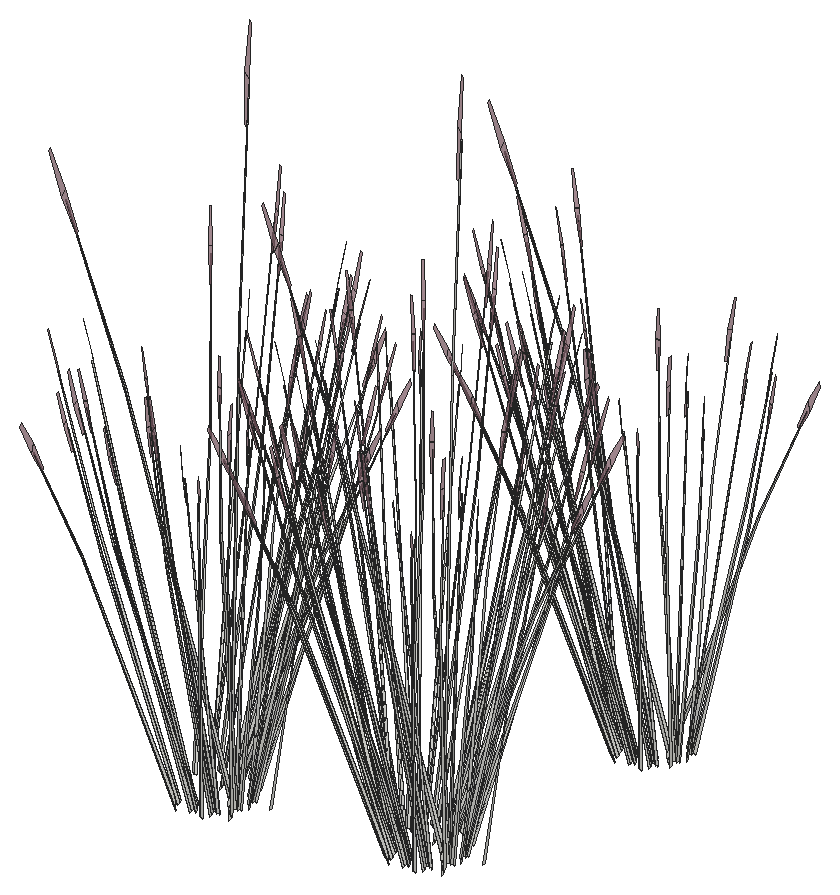
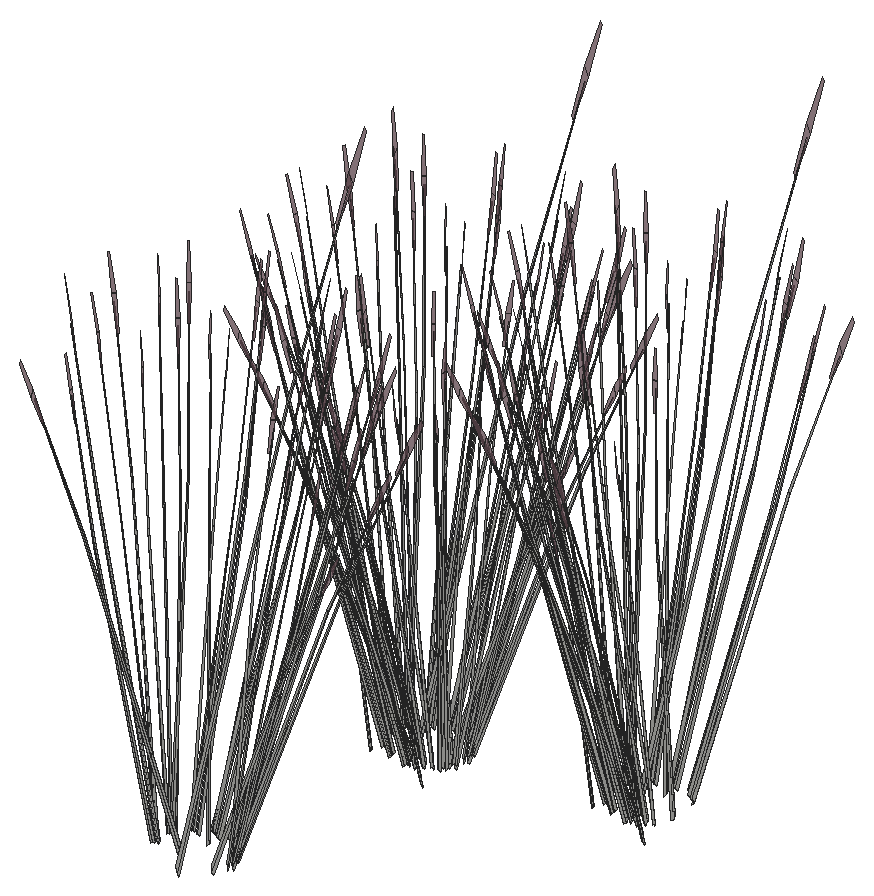
# SketchUp Ruby script. Lengths in inches.
U = 1.inch
M = Sketchup.active_model
def pt(a) = Geom::Point3d.new(a.map { |v| v * U })
def face(e, loops, mat)
  f = e.add_face(loops[0].map { |a| pt(a) })
  loops[1..].each { |l| e.add_face(l.map { |a| pt(a) }).erase! }
  f.material = f.back_material = mat if mat
  f
end
# faces: each face lists its corners as indices into pts; further lists are holes
def faces(e, pts, list, mat = nil) = list.each { |f| face(e, (f[0].is_a?(Array) ? f : [f]).map { |l| l.map { |i| pts[i] } }, mat) }
# xy, xz, yz: faces in a plane at the given z, y or x. An outline is a flat list of corners, or four numbers for a rectangle; further outlines are holes
def ring(l) = l.size == 4 ? [[l[0], l[1]], [l[2], l[1]], [l[2], l[3]], [l[0], l[3]]] : l.each_slice(2).to_a
def flat(e, list, mat, &to3) = list.each { |f| face(e, (f[0].is_a?(Array) ? f : [f]).map { |l| ring(l).map { |u, v| to3.(u, v) } }, mat) }
def xy(e, z, list, mat = nil) = flat(e, list, mat) { |x, y| [x, y, z] }
def xz(e, y, list, mat = nil) = flat(e, list, mat) { |x, z| [x, y, z] }
def yz(e, x, list, mat = nil) = flat(e, list, mat) { |y, z| [x, y, z] }
def lines(e, pts, list) = list.each { |a, b| e.add_line(pt(pts[a]), pt(pts[b])) }
# prism: a flat outline (further loops are holes) pulled along v
def prism(e, loops, v, mat = nil)
  f = face(e, loops, mat); d = Geom::Vector3d.new(v.map { |x| x * U })
  f.pushpull(f.normal.samedirection?(d) ? d.length : -d.length)
end
def box(e, o, s, mat = nil) = prism(e, [[o, [o[0] + s[0], o[1], o[2]], [o[0] + s[0], o[1] + s[1], o[2]], [o[0], o[1] + s[1], o[2]]]], [0, 0, s[2]], mat)
def at(x, y, z, deg = 0) = Geom::Transformation.translation(pt([x, y, z])) * Geom::Transformation.rotation(ORIGIN, Z_AXIS, deg.degrees)
def axes(o, x, y, z) = Geom::Transformation.new([*x, 0, *y, 0, *z, 0, *pt(o).to_a, 1])
def part(name) = M.definitions.add(name)
# library, detail: a bought-in or finely detailed component or shape, given as its bounding box
def library(name, o, s) = part(name).tap { |d| box(d.entities, o, s) }
def detail(e, o, s) = box(e.add_group.entities, o, s)
def put(e, d, t, mat = nil) = e.add_instance(d, t).tap { |i| i.material = mat if mat }
def group(e, t, mat = nil) = e.add_group.tap { |g| g.transformation = t; g.material = mat if mat }.entities
root = M.entities
M.materials.add("LightPink_Translucent").color = [144, 107, 117]
M.materials["LightPink_Translucent"].alpha = 0.75
c1 = part("blade")
p = [[2.15,0.21,22],[0,0.17,0],[0.09,0.45,0],[2.18,0.31,22],[2.29,0.31,22],[0.38,0.45,0],
  [2.48,0.24,33],[2.49,0.24,33],[2.48,0.22,33]]
faces(c1.entities,p,[[0,1,2,3],[4,5,2,3],[6,3,4,7],[8,0,3,6]])
c2 = part("seeds")
p = [[0.3,-0.1,1.38],[-0.01,-0.03,1.59],[-0.01,-0.03,0.03],[0.14,-0.07,-0.07],[0.29,-0.03,3],[0.15,0.01,3.11]]
faces(c2.entities,p,[[0,1,2,3],[1,0,4,5]],"LightPink_Translucent")
c3 = part("blade with seeds")
put(c3.entities,c1,at(0,0,0))
put(c3.entities,c2,axes([2.4,0.25,30.99],[1.5799,-0.05474,1.17369],[-0.12525,1.92788,0.29478],[-0.07173,-0.02425,1.56792]))
put(root,c3,axes([318.13,55.2,268.36],[-0.50465,0.12921,-0.47583],[-0.08828,-0.48932,-0.36857],[-0.13555,-0.14022,0.91046]))
put(root,c3,axes([316.91,57.76,268.6875],[0.47307,0.29971,-0.11324],[-0.27254,0.43404,-0.62851],[-0.13365,0.15087,0.95501]))
put(root,c3,axes([317.99,54.93,267.61],[0.1169,0.17452,1.59586],[-0.54019,0.14692,0.12904],[-0.12209,-0.27397,0.68222]))
put(root,c3,axes([318.18,54.83,268.22],[-0.07899,-0.43781,-0.32977],[0.45153,-0.11561,0.42575],[-0.12128,-0.12546,0.81462]))
put(root,c3,axes([317.5625,59.09,268.22],[-0.34603,0.28618,-0.32977],[-0.32756,-0.32677,0.42575],[-0.04984,0.16603,0.81462]))
put(root,c3,axes([319.375,58.15,267.1],[0.44194,0.21918,1.40854],[-0.43295,0.47219,0.557],[-0.19393,-0.27986,1.18082]))
put(root,c3,axes([317.79,58.79,268.97],[-0.01331,0.50278,-0.73435],[-0.56035,-0.03377,0.08862],[-0.05914,0.213,1.03881]))
put(root,c3,axes([317.6,59.5,267.13],[0.01124,-0.2806,1.43727],[0.50537,0.14821,0.19862],[-0.04379,0.29905,0.67868]))
put(root,c3,axes([317.91,58.95,268.66],[0.3661,0.36521,-0.52818],[-0.38674,0.31985,-0.40911],[-0.0557,0.18556,1.01061]))
put(root,c3,axes([320.0625,57.11,266.65],[-0.01397,-0.51177,1.31553],[0.63227,0.13266,0.557],[-0.14954,0.28003,1.24175]))
put(root,c3,axes([319.68,54.95,268.6875],[-0.50045,0.25306,-0.11324],[-0.24593,-0.44915,-0.62851],[-0.06603,-0.18927,0.95501]))
put(root,c3,axes([319.25,54.97,268.36],[-0.50273,-0.13626,-0.47583],[0.17232,-0.46717,-0.36857],[-0.0461,-0.18809,0.91046]))
put(root,c3,axes([318.32,58.43,267.61],[-0.01252,-0.20862,1.59586],[0.54251,0.1384,0.12904],[-0.03356,0.2973,0.68222]))
put(root,c3,axes([319.43,55.06,268.64],[-0.24409,-0.44196,-0.66157],[0.50245,-0.2463,0.07984],[-0.05708,-0.21354,0.93586]))
put(root,c3,axes([319.48,54.68,268.22],[0.15418,-0.41799,-0.32977],[0.44981,0.12192,0.42575],[-0.04124,-0.16829,0.81462]))
put(root,c3,axes([318.76,59.59,268.22],[-0.15418,0.41799,-0.32977],[-0.44981,-0.12192,0.42575],[0.04124,0.16829,0.81462]))
put(root,c3,axes([318.81,59.22,268.64],[0.24409,0.44196,-0.66157],[-0.50245,0.2463,0.07984],[0.05708,0.21354,0.93586]))
put(root,c3,axes([318.99,59.31,268.36],[0.50273,0.13626,-0.47583],[-0.17232,0.46717,-0.36857],[0.0461,0.18809,0.91046]))
put(root,c3,axes([318.5625,59.33,268.6875],[0.50045,-0.25306,-0.11324],[0.24593,0.44915,-0.62851],[0.06603,0.18927,0.95501]))
put(root,c3,axes([320.72,55.51,268.6875],[-0.56206,-0.02693,-0.11324],[0.01536,-0.50991,-0.62851],[0.03904,-0.19638,0.95501]))
put(root,c3,axes([320.34,55.32,268.36],[-0.3661,-0.36521,-0.47583],[0.38674,-0.31985,-0.36857],[0.0557,-0.18556,0.91046]))
put(root,c3,axes([319.28,58.34,267.61],[-0.1169,-0.17452,1.59586],[0.54019,-0.14692,0.12904],[0.12209,0.27397,0.68222]))
put(root,c3,axes([320.45,55.49,268.64],[0.01331,-0.50278,-0.66157],[0.56035,0.03377,0.07984],[0.05914,-0.213,0.93586]))
put(root,c3,axes([320.68,55.1875,268.22],[0.34603,-0.28618,-0.32977],[0.32756,0.32677,0.42575],[0.04984,-0.16603,0.81462]))
put(root,c3,axes([319.82,55.23,267.61],[-0.09522,0.18683,1.59586],[-0.39947,-0.38663,0.12904],[0.18021,-0.24097,0.68222]))
put(root,c3,axes([319.75,59.3125,268.6875],[0.30474,-0.46525,-0.11324],[0.44133,0.26804,-0.62851],[0.15341,0.13145,0.95501]))
put(root,c3,axes([321.33,56.52,268.6875],[-0.47307,-0.29971,-0.11324],[0.27254,-0.43404,-0.62851],[0.13365,-0.15087,0.95501]))
put(root,c3,axes([320.11,59.08,268.36],[0.50465,-0.12921,-0.47583],[0.08828,0.48932,-0.36857],[0.13555,0.14022,0.91046]))
put(root,c3,axes([321.1,56.16,268.36],[-0.13138,-0.49631,-0.47583],[0.49754,-0.08682,-0.36857],[0.14258,-0.13331,0.91046]))
put(root,c3,axes([321.97,58.72,267.66],[-0.09788,-0.45691,-0.03251],[0.46264,-0.10504,-0.14742],[0.09661,0.02897,0.48626]))
put(root,c3,axes([320.06,57.8,267.61],[-0.18996,-0.09365,1.59586],[0.39312,-0.39287,0.12904],[0.24502,0.17723,0.68222]))
put(root,c3,axes([321.46,56.22,268.22],[0.44516,-0.07768,-0.32977],[0.11755,0.44407,0.42575],[0.12757,-0.11927,0.81462]))
put(root,c3,axes([321.11,56.36,268.64],[0.26714,-0.42887,-0.66157],[0.46811,0.30479,0.07984],[0.1595,-0.15539,0.93586]))
put(root,c3,axes([321.1,58.67,268.22],[0.29098,0.34031,-0.32977],[-0.33226,0.32215,0.42575],[0.16881,0.04902,0.81462]))
put(root,c3,axes([320.77,58.71,268.6875],[0.02738,-0.55277,-0.11324],[0.51847,0.01511,-0.62851],[0.19968,0.0384,0.95501]))
put(root,c3,axes([321.35,57.6875,268.6875],[-0.25732,-0.49218,-0.11324],[0.45669,-0.24187,-0.62851],[0.19245,-0.06494,0.95501]))
put(root,c3,axes([321.33,57.26,268.36],[0.13855,-0.49442,-0.47583],[0.47502,0.16947,-0.36857],[0.19125,-0.04534,0.91046]))
put(root,c3,axes([321.62,57.49,268.22],[0.42502,0.15163,-0.32977],[-0.12396,0.44238,0.42575],[0.17112,-0.04056,0.81462]))
put(root,c3,axes([330.64,59.02,267.61],[0.21212,-0.01231,1.59586],[-0.14072,0.53355,0.12904],[-0.3023,-0.033,0.68222]))
put(root,c3,axes([320.8,58.44,268.64],[0.51122,0.01309,-0.66157],[-0.03434,0.5511,0.07984],[0.21658,0.05816,0.93586]))
put(root,c3,axes([320.46,56.94,267.61],[-0.21212,0.01231,1.59586],[0.14072,-0.53355,0.12904],[0.3023,0.033,0.68222]))
put(root,c3,axes([321.24,57.45,268.64],[0.44939,-0.24006,-0.66157],[0.25044,0.49415,0.07984],[0.21713,-0.05613,0.93586]))
put(root,c3,axes([330.73,59.96,267.61],[0.17745,-0.11497,1.59586],[0.14939,0.53127,0.12904],[-0.27857,0.12007,0.68222]))
put(root,c3,axes([331.75,59.41,267.11],[0.14537,-0.07863,1.64882],[0.05013,0.549,0.12904],[-0.31487,0.07285,0.5893]))
put(root,c3,axes([331.28,58.53,268.64],[-0.51122,-0.01309,-0.66157],[0.03434,-0.5511,0.07984],[-0.21658,-0.05816,0.93586]))
put(root,c3,axes([330.46,59.48,268.22],[-0.42502,-0.15163,-0.32977],[0.12396,-0.44238,0.42575],[-0.17112,0.04056,0.81462]))
put(root,c3,axes([331.04,58.17,267.61],[0.18996,0.09365,1.59586],[-0.39312,0.39287,0.12904],[-0.24502,-0.17723,0.68222]))
put(root,c3,axes([330.75,59.71,268.36],[-0.13855,0.49442,-0.47583],[-0.47502,-0.16947,-0.36857],[-0.19125,0.04534,0.91046]))
put(root,c3,axes([331.11,58.64,268.36],[-0.37135,0.36005,-0.47583],[-0.32522,-0.38035,-0.36857],[-0.18868,-0.05478,0.91046]))
put(root,c3,axes([330.72,59.29,268.6875],[0.25732,0.49218,-0.11324],[-0.45669,0.24187,-0.62851],[-0.19245,0.06494,0.95501]))
put(root,c3,axes([331.3,58.26,268.6875],[-0.02738,0.55277,-0.11324],[-0.51847,-0.01511,-0.62851],[-0.19968,-0.0384,0.95501]))
put(root,c3,axes([330.97,58.3,268.22],[-0.29098,-0.34031,-0.32977],[0.33226,-0.32215,0.42575],[-0.16881,-0.04902,0.81462]))
put(root,c3,axes([331.38,60.32,267.61],[0.12773,-0.16701,1.59586],[0.32252,0.4508,0.12904],[-0.22121,0.20529,0.68222]))
put(root,c3,axes([330.61,60.76,268.22],[-0.44516,0.07768,-0.32977],[-0.11755,-0.44407,0.42575],[-0.12757,0.11927,0.81462]))
put(root,c3,axes([333.34,76.875,267.61],[0.21212,-0.01231,1.59586],[-0.14072,0.53355,0.12904],[-0.3023,-0.033,0.68222]))
put(root,c3,axes([331.28,60.73,267.61],[0.09522,-0.18683,1.59586],[0.39947,0.38663,0.12904],[-0.18021,0.24097,0.68222]))
put(root,c3,axes([330.98,60.81,268.36],[0.13138,0.49631,-0.47583],[-0.49754,0.08682,-0.36857],[-0.14258,0.13331,0.91046]))
put(root,c3,axes([332.17,57.88,268.64],[-0.43608,-0.26272,-0.66157],[0.30991,-0.46038,0.07984],[-0.158,-0.15687,0.93586]))
put(root,c3,axes([331.96,57.89,268.36],[-0.50465,0.12921,-0.47583],[-0.08828,-0.48932,-0.36857],[-0.13555,-0.14022,0.91046]))
put(root,c3,axes([330.74,60.46,268.6875],[0.47307,0.29971,-0.11324],[-0.27254,0.43404,-0.62851],[-0.13365,0.15087,0.95501]))
put(root,c3,axes([334.45,77.26,267.11],[0.14537,-0.07863,1.64882],[0.05013,0.549,0.12904],[-0.31487,0.07285,0.5893]))
put(root,c3,axes([333.97,76.38,268.64],[-0.51122,-0.01309,-0.66157],[0.03434,-0.5511,0.07984],[-0.21658,-0.05816,0.93586]))
put(root,c3,axes([333.15,77.33,268.22],[-0.42502,-0.15163,-0.32977],[0.12396,-0.44238,0.42575],[-0.17112,0.04056,0.81462]))
put(root,c3,axes([333.74,76.02,267.61],[0.18996,0.09365,1.59586],[-0.39312,0.39287,0.12904],[-0.24502,-0.17723,0.68222]))
put(root,c3,axes([331.83,57.625,267.61],[0.1169,0.17452,1.59586],[-0.54019,0.14692,0.12904],[-0.12209,-0.27397,0.68222]))
put(root,c3,axes([333.44,77.56,268.36],[-0.13855,0.49442,-0.47583],[-0.47502,-0.16947,-0.36857],[-0.19125,0.04534,0.91046]))
put(root,c3,axes([333.8,76.49,268.36],[-0.37135,0.36005,-0.47583],[-0.32522,-0.38035,-0.36857],[-0.18868,-0.05478,0.91046]))
put(root,c3,axes([332.01,57.53,268.22],[-0.07899,-0.43781,-0.32977],[0.45153,-0.11561,0.42575],[-0.12128,-0.12546,0.81462]))
put(root,c3,axes([331.39,61.79,268.22],[-0.34603,0.28618,-0.32977],[-0.32756,-0.32677,0.42575],[-0.04984,0.16603,0.81462]))
put(root,c3,axes([333.42,77.13,268.6875],[0.25732,0.49218,-0.11324],[-0.45669,0.24187,-0.62851],[-0.19245,0.06494,0.95501]))
put(root,c3,axes([334,76.11,268.6875],[-0.02738,0.55277,-0.11324],[-0.51847,-0.01511,-0.62851],[-0.19968,-0.0384,0.95501]))
put(root,c3,axes([333.21,60.85,267.1],[0.44194,0.21918,1.40854],[-0.43295,0.47219,0.557],[-0.19393,-0.27986,1.18082]))
put(root,c3,axes([333.67,76.15,268.22],[-0.29098,-0.34031,-0.32977],[0.33226,-0.32215,0.42575],[-0.16881,-0.04902,0.81462]))
put(root,c3,axes([331.625,61.48,268.97],[-0.01331,0.50278,-0.73435],[-0.56035,-0.03377,0.08862],[-0.05914,0.213,1.03881]))
put(root,c3,axes([331.4375,62.19,267.13],[0.01124,-0.2806,1.43727],[0.50537,0.14821,0.19862],[-0.04379,0.29905,0.67868]))
put(root,c3,axes([331.74,61.65,268.66],[0.3661,0.36521,-0.52818],[-0.38674,0.31985,-0.40911],[-0.0557,0.18556,1.01061]))
put(root,c3,axes([333.89,59.8,266.65],[-0.01397,-0.51177,1.31553],[0.63227,0.13266,0.557],[-0.14954,0.28003,1.24175]))
put(root,c3,axes([334.86,75.73,268.64],[-0.43608,-0.26272,-0.66157],[0.30991,-0.46038,0.07984],[-0.158,-0.15687,0.93586]))
put(root,c3,axes([334.66,75.74,268.36],[-0.50465,0.12921,-0.47583],[-0.08828,-0.48932,-0.36857],[-0.13555,-0.14022,0.91046]))
put(root,c3,axes([333.51,57.64,268.6875],[-0.50045,0.25306,-0.11324],[-0.24593,-0.44915,-0.62851],[-0.06603,-0.18927,0.95501]))
put(root,c3,axes([333.08,57.67,268.36],[-0.50273,-0.13626,-0.47583],[0.17232,-0.46717,-0.36857],[-0.0461,-0.18809,0.91046]))
put(root,c3,axes([332.15,61.13,267.61],[-0.01252,-0.20862,1.59586],[0.54251,0.1384,0.12904],[-0.03356,0.2973,0.68222]))
put(root,c3,axes([333.27,57.75,268.64],[-0.24409,-0.44196,-0.66157],[0.50245,-0.2463,0.07984],[-0.05708,-0.21354,0.93586]))
put(root,c3,axes([334.52,75.47,267.61],[0.1169,0.17452,1.59586],[-0.54019,0.14692,0.12904],[-0.12209,-0.27397,0.68222]))
put(root,c3,axes([334.71,75.38,268.22],[-0.07899,-0.43781,-0.32977],[0.45153,-0.11561,0.42575],[-0.12128,-0.12546,0.81462]))
put(root,c3,axes([333.3125,57.38,268.22],[0.15418,-0.41799,-0.32977],[0.44981,0.12192,0.42575],[-0.04124,-0.16829,0.81462]))
put(root,c3,axes([335.91,78.7,267.1],[0.44194,0.21918,1.40854],[-0.43295,0.47219,0.557],[-0.19393,-0.27986,1.18082]))
put(root,c3,axes([332.59,62.29,268.22],[-0.15418,0.41799,-0.32977],[-0.44981,-0.12192,0.42575],[0.04124,0.16829,0.81462]))
put(root,c3,axes([332.64,61.92,268.64],[0.24409,0.44196,-0.66157],[-0.50245,0.2463,0.07984],[0.05708,0.21354,0.93586]))
put(root,c3,axes([336.21,75.49,268.6875],[-0.50045,0.25306,-0.11324],[-0.24593,-0.44915,-0.62851],[-0.06603,-0.18927,0.95501]))
put(root,c3,axes([335.78,75.51,268.36],[-0.50273,-0.13626,-0.47583],[0.17232,-0.46717,-0.36857],[-0.0461,-0.18809,0.91046]))
put(root,c3,axes([332.82,62.01,268.36],[0.50273,0.13626,-0.47583],[-0.17232,0.46717,-0.36857],[0.0461,0.18809,0.91046]))
put(root,c3,axes([332.39,62.03,268.6875],[0.50045,-0.25306,-0.11324],[0.24593,0.44915,-0.62851],[0.06603,0.18927,0.95501]))
put(root,c3,axes([334.55,58.21,268.6875],[-0.56206,-0.02693,-0.11324],[0.01536,-0.50991,-0.62851],[0.03904,-0.19638,0.95501]))
put(root,c3,axes([335.96,75.6,268.64],[-0.24409,-0.44196,-0.66157],[0.50245,-0.2463,0.07984],[-0.05708,-0.21354,0.93586]))
put(root,c3,axes([334.17,58.02,268.36],[-0.3661,-0.36521,-0.47583],[0.38674,-0.31985,-0.36857],[0.0557,-0.18556,0.91046]))
put(root,c3,axes([333.11,61.04,267.61],[-0.1169,-0.17452,1.59586],[0.54019,-0.14692,0.12904],[0.12209,0.27397,0.68222]))
put(root,c3,axes([334.28,58.1875,268.64],[0.01331,-0.50278,-0.66157],[0.56035,0.03377,0.07984],[0.05914,-0.213,0.93586]))
put(root,c3,axes([336.01,75.23,268.22],[0.15418,-0.41799,-0.32977],[0.44981,0.12192,0.42575],[-0.04124,-0.16829,0.81462]))
put(root,c3,axes([334.51,57.88,268.22],[0.34603,-0.28618,-0.32977],[0.32756,0.32677,0.42575],[0.04984,-0.16603,0.81462]))
put(root,c3,axes([333.65,57.93,267.61],[-0.09522,0.18683,1.59586],[-0.39947,-0.38663,0.12904],[0.18021,-0.24097,0.68222]))
put(root,c3,axes([333.58,62.01,268.6875],[0.30474,-0.46525,-0.11324],[0.44133,0.26804,-0.62851],[0.15341,0.13145,0.95501]))
put(root,c3,axes([335.16,59.21,268.6875],[-0.47307,-0.29971,-0.11324],[0.27254,-0.43404,-0.62851],[0.13365,-0.15087,0.95501]))
put(root,c3,axes([333.94,61.78,268.36],[0.50465,-0.12921,-0.47583],[0.08828,0.48932,-0.36857],[0.13555,0.14022,0.91046]))
put(root,c3,axes([337.25,76.0625,268.6875],[-0.56206,-0.02693,-0.11324],[0.01536,-0.50991,-0.62851],[0.03904,-0.19638,0.95501]))
put(root,c3,axes([334.93,58.86,268.36],[-0.13138,-0.49631,-0.47583],[0.49754,-0.08682,-0.36857],[0.14258,-0.13331,0.91046]))
put(root,c3,axes([336.86,75.87,268.36],[-0.3661,-0.36521,-0.47583],[0.38674,-0.31985,-0.36857],[0.0557,-0.18556,0.91046]))
put(root,c3,axes([335.8,61.42,267.66],[-0.09788,-0.45691,-0.03251],[0.46264,-0.10504,-0.14742],[0.09661,0.02897,0.48626]))
put(root,c3,axes([333.89,60.5,267.61],[-0.18996,-0.09365,1.59586],[0.39312,-0.39287,0.12904],[0.24502,0.17723,0.68222]))
put(root,c3,axes([336.98,76.04,268.64],[0.01331,-0.50278,-0.66157],[0.56035,0.03377,0.07984],[0.05914,-0.213,0.93586]))
put(root,c3,axes([335.3,58.91,268.22],[0.44516,-0.07768,-0.32977],[0.11755,0.44407,0.42575],[0.12757,-0.11927,0.81462]))
put(root,c3,axes([334.94,59.06,268.64],[0.26714,-0.42887,-0.66157],[0.46811,0.30479,0.07984],[0.1595,-0.15539,0.93586]))
put(root,c3,axes([334.9375,61.37,268.22],[0.29098,0.34031,-0.32977],[-0.33226,0.32215,0.42575],[0.16881,0.04902,0.81462]))
put(root,c3,axes([334.6,61.41,268.6875],[0.02738,-0.55277,-0.11324],[0.51847,0.01511,-0.62851],[0.19968,0.0384,0.95501]))
put(root,c3,axes([335.18,60.38,268.6875],[-0.25732,-0.49218,-0.11324],[0.45669,-0.24187,-0.62851],[0.19245,-0.06494,0.95501]))
put(root,c3,axes([337.21,75.73,268.22],[0.34603,-0.28618,-0.32977],[0.32756,0.32677,0.42575],[0.04984,-0.16603,0.81462]))
put(root,c3,axes([335.16,59.96,268.36],[0.13855,-0.49442,-0.47583],[0.47502,0.16947,-0.36857],[0.19125,-0.04534,0.91046]))
put(root,c3,axes([335.45,60.1875,268.22],[0.42502,0.15163,-0.32977],[-0.12396,0.44238,0.42575],[0.17112,-0.04056,0.81462]))
put(root,c3,axes([334.63,61.14,268.64],[0.51122,0.01309,-0.66157],[-0.03434,0.5511,0.07984],[0.21658,0.05816,0.93586]))
put(root,c3,axes([336.35,75.78,267.61],[-0.09522,0.18683,1.59586],[-0.39947,-0.38663,0.12904],[0.18021,-0.24097,0.68222]))
put(root,c3,axes([334.29,59.64,267.61],[-0.21212,0.01231,1.59586],[0.14072,-0.53355,0.12904],[0.3023,0.033,0.68222]))
put(root,c3,axes([337.86,77.0625,268.6875],[-0.47307,-0.29971,-0.11324],[0.27254,-0.43404,-0.62851],[0.13365,-0.15087,0.95501]))
put(root,c3,axes([335.07,60.14,268.64],[0.44939,-0.24006,-0.66157],[0.25044,0.49415,0.07984],[0.21713,-0.05613,0.93586]))
put(root,c3,axes([337.625,76.71,268.36],[-0.13138,-0.49631,-0.47583],[0.49754,-0.08682,-0.36857],[0.14258,-0.13331,0.91046]))
put(root,c3,axes([337.99,76.76,268.22],[0.44516,-0.07768,-0.32977],[0.11755,0.44407,0.42575],[0.12757,-0.11927,0.81462]))
put(root,c3,axes([337.64,76.91,268.64],[0.26714,-0.42887,-0.66157],[0.46811,0.30479,0.07984],[0.1595,-0.15539,0.93586]))
put(root,c3,axes([337.88,78.23,268.6875],[-0.25732,-0.49218,-0.11324],[0.45669,-0.24187,-0.62851],[0.19245,-0.06494,0.95501]))
put(root,c3,axes([337.86,77.8125,268.36],[0.13855,-0.49442,-0.47583],[0.47502,0.16947,-0.36857],[0.19125,-0.04534,0.91046]))
put(root,c3,axes([338.15,78.04,268.22],[0.42502,0.15163,-0.32977],[-0.12396,0.44238,0.42575],[0.17112,-0.04056,0.81462]))
put(root,c3,axes([336.99,77.49,267.61],[-0.21212,0.01231,1.59586],[0.14072,-0.53355,0.12904],[0.3023,0.033,0.68222]))
put(root,c3,axes([337.77,77.99,268.64],[0.44939,-0.24006,-0.66157],[0.25044,0.49415,0.07984],[0.21713,-0.05613,0.93586]))
